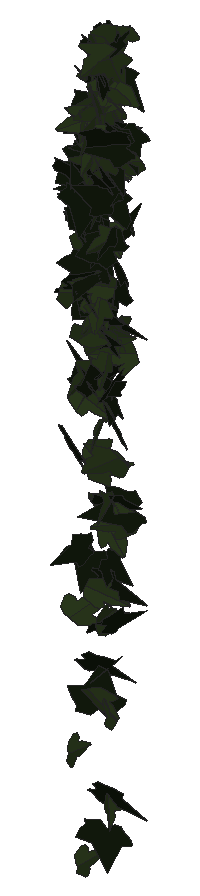
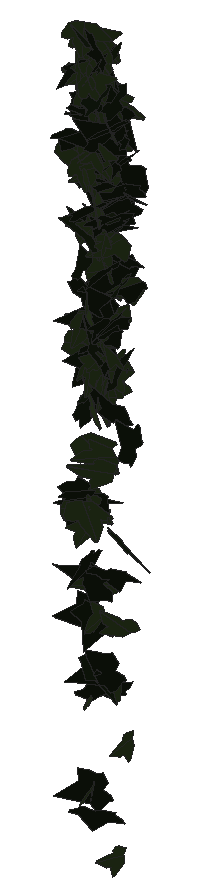
# SketchUp Ruby script. Lengths in inches.
U = 1.inch
M = Sketchup.active_model
def pt(a) = Geom::Point3d.new(a.map { |v| v * U })
def face(e, loops, mat)
  f = e.add_face(loops[0].map { |a| pt(a) })
  loops[1..].each { |l| e.add_face(l.map { |a| pt(a) }).erase! }
  f.material = f.back_material = mat if mat
  f
end
# faces: each face lists its corners as indices into pts; further lists are holes
def faces(e, pts, list, mat = nil) = list.each { |f| face(e, (f[0].is_a?(Array) ? f : [f]).map { |l| l.map { |i| pts[i] } }, mat) }
# xy, xz, yz: faces in a plane at the given z, y or x. An outline is a flat list of corners, or four numbers for a rectangle; further outlines are holes
def ring(l) = l.size == 4 ? [[l[0], l[1]], [l[2], l[1]], [l[2], l[3]], [l[0], l[3]]] : l.each_slice(2).to_a
def flat(e, list, mat, &to3) = list.each { |f| face(e, (f[0].is_a?(Array) ? f : [f]).map { |l| ring(l).map { |u, v| to3.(u, v) } }, mat) }
def xy(e, z, list, mat = nil) = flat(e, list, mat) { |x, y| [x, y, z] }
def xz(e, y, list, mat = nil) = flat(e, list, mat) { |x, z| [x, y, z] }
def yz(e, x, list, mat = nil) = flat(e, list, mat) { |y, z| [x, y, z] }
def lines(e, pts, list) = list.each { |a, b| e.add_line(pt(pts[a]), pt(pts[b])) }
# prism: a flat outline (further loops are holes) pulled along v
def prism(e, loops, v, mat = nil)
  f = face(e, loops, mat); d = Geom::Vector3d.new(v.map { |x| x * U })
  f.pushpull(f.normal.samedirection?(d) ? d.length : -d.length)
end
def box(e, o, s, mat = nil) = prism(e, [[o, [o[0] + s[0], o[1], o[2]], [o[0] + s[0], o[1] + s[1], o[2]], [o[0], o[1] + s[1], o[2]]]], [0, 0, s[2]], mat)
def at(x, y, z, deg = 0) = Geom::Transformation.translation(pt([x, y, z])) * Geom::Transformation.rotation(ORIGIN, Z_AXIS, deg.degrees)
def axes(o, x, y, z) = Geom::Transformation.new([*x, 0, *y, 0, *z, 0, *pt(o).to_a, 1])
def part(name) = M.definitions.add(name)
# library, detail: a bought-in or finely detailed component or shape, given as its bounding box
def library(name, o, s) = part(name).tap { |d| box(d.entities, o, s) }
def detail(e, o, s) = box(e.add_group.entities, o, s)
def put(e, d, t, mat = nil) = e.add_instance(d, t).tap { |i| i.material = mat if mat }
def group(e, t, mat = nil) = e.add_group.tap { |g| g.transformation = t; g.material = mat if mat }.entities
root = M.entities
M.materials.add("1026 AP 7946 SUNNY SIDE UP").color = [254, 231, 186]
M.materials.add("efeu1").color = [18, 25, 13]
M.materials.add("efeu2").color = [43, 57, 29]
c1 = part("ivyleaf_10")
p = [[0,0.5,-0.03],[-0.0625,2.02,-0.43],[-0.19,2.01,-0.46],[-0.54,1.05,-0.29],[-0.52,0.625,-0.18],[-0.83,0.76,-0.28],
  [-1.16,0.64,-0.33],[-1.15,0.33,-0.24],[-0.77,-0.39,0.02],[-0.3,-0.51,0.16],[0.04,-0.48,0.23],[-0.02,2.01,-0.4375],
  [-0.06,2.01,-0.43],[0.04,-0.49,0.23],[0.67,-0.49,0.14],[1.38,0.36,-0.2],[1.375,0.51,-0.24],[0.81,0.65,-0.19],
  [0.62,0.59,-0.15],[0.6,1.09,-0.28],[0.5,1.23,-0.31]]
faces(c1.entities,p,[[0,1,2,3,4,5,6,7,8,9,10],[11,12,0,13,14,15,16,17,18,19,20]],"efeu2")
c2 = part("ivyleaf_9")
p = [[1.54,2.16,1.25],[1.36,2.04,1.19],[-0.21,0.99,0.68],[-0.71,1.11,0.82],[-0.85,0.86,0.67],[-0.8,0.17,0.21],
  [-0.9,-0.01,0.1],[-0.67,-0.16,-0.02],[-0.08,-0.08,-0.05],[-0.03,-0.6,-0.4],[0.65,-0.88,-0.66],[0.83,-0.6,-0.49],
  [1.29,-0.42,-0.43],[1.8125,-0.07,-0.26],[1.21,0.44,0.15]]
faces(c2.entities,p,[[0,1,2,3,4,5,6,7,8,9,10,11,12,13,14]],"efeu1")
put(root,c1,axes([111.49,212.18,255.23],[0.26349,0.05357,-0.16919],[0.22588,0.08462,0.1796],[0.15168,-0.21907,0.02645]),"1026 AP 7946 SUNNY SIDE UP")
put(root,c2,axes([111.56,212.58,265.79],[-0.01777,-0.25367,-0.01098],[0.00914,0.00897,-0.26147],[0.39902,-0.0115,0.0055]),"1026 AP 7946 SUNNY SIDE UP")
put(root,c2,axes([111.58,212.3125,264.45],[-0.15826,-0.2049,-0.12442],[0.09307,0.10414,-0.23447],[0.36127,-0.11658,0.0059]),"1026 AP 7946 SUNNY SIDE UP")
put(root,c2,axes([111.5,212.4,265.18],[0.21603,-0.20442,-0.0599],[-0.03502,0.05362,-0.25316],[0.33184,0.13874,0.01228]),"1026 AP 7946 SUNNY SIDE UP")
put(root,c1,axes([111.69,212.07,264.54],[0.1941,-0.22333,0.03277],[0.00495,-0.03599,-0.26266],[0.35495,0.12263,-0.01426]),"1026 AP 7946 SUNNY SIDE UP")
put(root,c1,axes([111.73,212.0625,265.4],[-0.09146,0.18682,0.15912],[-0.11423,0.13697,-0.19943],[-0.36252,-0.09029,0.02269]),"1026 AP 7946 SUNNY SIDE UP")
put(root,c2,axes([111.5,212.48,259.78],[-0.1363,0.1013,0.21327],[0.24989,-0.13307,0.13523],[0.26134,0.18007,-0.01808]),"1026 AP 7946 SUNNY SIDE UP")
put(root,c2,axes([111.5625,212.44,261.74],[0.14333,-0.20924,-0.0936],[-0.06701,0.0792,-0.23455],[0.35162,0.10039,-0.00654]),"1026 AP 7946 SUNNY SIDE UP")
put(root,c2,axes([111.55,212.14,263.63],[0.15097,-0.22676,-0.03682],[-0.04058,0.02643,-0.25316],[0.35836,0.09852,-0.01316]),"1026 AP 7946 SUNNY SIDE UP")
put(root,c2,axes([111.43,211.99,258.95],[0.22206,-0.06541,-0.22293],[0.32923,-0.05721,0.15852],[-0.13255,-0.25167,0.02026]),"1026 AP 7946 SUNNY SIDE UP")
put(root,c2,axes([111.45,212.45,266.36],[0.29605,-0.16673,0.0648],[0.05532,-0.05632,-0.25873],[0.27523,0.19067,-0.0177]),"1026 AP 7946 SUNNY SIDE UP")
put(root,c2,axes([111.75,212.18,263.86],[0.31124,-0.00117,0.1752],[-0.26329,0.04437,0.20134],[-0.04685,-0.25717,0.03239]),"1026 AP 7946 SUNNY SIDE UP")
put(root,c2,axes([111.6,212.4375,261.6875],[0.00784,-0.19578,-0.15333],[-0.00771,0.14765,-0.20089],[0.38557,0.00693,-0.0009]),"1026 AP 7946 SUNNY SIDE UP")
put(root,c1,axes([111.9,212.58,265.2],[-0.34377,-0.00563,0.1266],[-0.18522,-0.0629,-0.21917],[0.05595,-0.2428,0.05232]),"1026 AP 7946 SUNNY SIDE UP")
put(root,c2,axes([111.625,211.9375,264.7],[0.44384,0.05371,-0.09486],[-0.13287,-0.04753,-0.29473],[-0.10285,0.29318,-0.02859]),"1026 AP 7946 SUNNY SIDE UP")
put(root,c1,axes([111.57,211.8,262.16],[-0.03675,-0.05095,-0.23565],[0.23229,0.17488,-0.05473],[0.28549,-0.14885,0.0142]),"1026 AP 7946 SUNNY SIDE UP")
put(root,c2,axes([111.72,212.41,256.45],[-0.29436,-0.1468,-0.06734],[0.09721,0.02546,-0.24427],[0.23266,-0.19637,0.01686]),"1026 AP 7946 SUNNY SIDE UP")
put(root,c2,axes([111.6875,212.21,264.8],[-0.09378,-0.20137,0.14095],[-0.05911,-0.13274,-0.21713],[0.37924,-0.07048,0.00101]),"1026 AP 7946 SUNNY SIDE UP")
put(root,c1,axes([111.72,212.38,265.78],[0.18876,-0.21054,0.07497],[0.04092,-0.07021,-0.2498],[0.3485,0.12228,-0.01127]),"1026 AP 7946 SUNNY SIDE UP")
put(root,c2,axes([111.95,211.9,256.875],[-0.31961,0.12959,-0.02596],[0.01723,-0.0309,-0.24765],[-0.20709,-0.20257,0.01947]),"1026 AP 7946 SUNNY SIDE UP")
put(root,c2,axes([111.64,212.58,262.82],[0.07735,-0.23071,-0.0778],[-0.02575,0.07239,-0.24259],[0.38021,0.05184,-0.0006]),"1026 AP 7946 SUNNY SIDE UP")
put(root,c1,axes([111.83,212.25,266.01],[-0.07473,-0.23429,0.07325],[-0.00508,-0.07317,-0.24645],[0.38557,-0.04637,0.01095]),"1026 AP 7946 SUNNY SIDE UP")
put(root,c1,axes([111.74,211.75,252.61],[-0.00129,-0.04435,-0.2514],[0.09781,0.23594,-0.04306],[0.37714,-0.06134,0.01031]),"1026 AP 7946 SUNNY SIDE UP")
put(root,c1,axes([111.6875,212.46,261.11],[0.34374,-0.11681,0.10042],[0.11864,-0.06627,-0.25478],[0.2085,0.23028,-0.02058]),"1026 AP 7946 SUNNY SIDE UP")
put(root,c2,axes([111.67,212.35,263.78],[-0.05512,-0.23077,-0.12773],[0.04427,0.11972,-0.2396],[0.40855,-0.04411,0.00873]),"1026 AP 7946 SUNNY SIDE UP")
put(root,c2,axes([112,212.04,265.81],[0.11588,0.09421,-0.22902],[-0.28417,-0.13344,-0.12047],[-0.25292,0.19309,0.03042]),"1026 AP 7946 SUNNY SIDE UP")
put(root,c2,axes([111.93,212.14,260.21],[0.07343,-0.2493,0.13933],[-0.02013,0.13651,0.26185],[-0.44659,-0.04714,0.0111]),"1026 AP 7946 SUNNY SIDE UP")
put(root,c2,axes([111.5625,212.35,265.27],[0.14322,-0.14456,0.18881],[0.15484,-0.15555,-0.17693],[0.3339,0.13414,0.00106]),"1026 AP 7946 SUNNY SIDE UP")
put(root,c2,axes([111.7,212.4,265.43],[-0.07135,-0.02984,0.28062],[0.36249,0.14542,0.05679],[-0.23342,0.23495,0.00241]),"1026 AP 7946 SUNNY SIDE UP")
put(root,c1,axes([111.68,212.19,263.22],[-0.17067,-0.10762,-0.20235],[0.2606,0.10722,-0.15473],[0.23563,-0.19654,0.02456]),"1026 AP 7946 SUNNY SIDE UP")
put(root,c1,axes([111.8,212.07,260.42],[0.04402,-0.09335,0.29078],[0.12483,-0.27141,-0.10199],[0.4513,0.08418,-0.00015]),"1026 AP 7946 SUNNY SIDE UP")
put(root,c1,axes([112.03,211.96,265.89],[0.22377,0.05359,-0.2239],[-0.29814,-0.10871,-0.15593],[-0.18797,0.23623,-0.01922]),"1026 AP 7946 SUNNY SIDE UP")
put(root,c2,axes([111.76,212.02,264.05],[-0.06303,-0.24689,0.08918],[0.00151,-0.08913,-0.25777],[0.41212,-0.03743,0.01459]),"1026 AP 7946 SUNNY SIDE UP")
put(root,c2,axes([111.58,212.35,265.42],[0.21953,0.059,0.22804],[0.3316,0.06714,-0.15531],[-0.13939,0.25266,-0.01032]),"1026 AP 7946 SUNNY SIDE UP")
put(root,c1,axes([111.92,212.62,266.66],[-0.17471,-0.20305,0.11598],[-0.00404,-0.12495,-0.23313],[0.36593,-0.09832,0.0528]),"1026 AP 7946 SUNNY SIDE UP")
put(root,c2,axes([111.66,211.79,262.33],[0.26184,0.14155,0.21204],[0.26564,0.1171,-0.22396],[-0.28793,0.23675,-0.01379]),"1026 AP 7946 SUNNY SIDE UP")
put(root,c2,axes([111.79,212.38,267.13],[0.18853,-0.18165,-0.17069],[-0.14945,0.13452,-0.22339],[0.35536,0.15294,-0.00339]),"1026 AP 7946 SUNNY SIDE UP")
put(root,c2,axes([111.7,212.12,262.22],[0.17634,-0.23271,0.03459],[0.0087,-0.03604,-0.26611],[0.36991,0.11178,-0.01023]),"1026 AP 7946 SUNNY SIDE UP")
put(root,c1,axes([111.91,212.05,260.04],[0.00158,-0.22037,-0.1156],[0.03959,0.11047,-0.22515],[0.38594,-0.01043,0.02357]),"1026 AP 7946 SUNNY SIDE UP")
put(root,c2,axes([112.21,212.3,264.34],[-0.35931,0.03377,0.14084],[-0.21935,-0.02139,-0.23522],[-0.02805,-0.26533,0.0353]),"1026 AP 7946 SUNNY SIDE UP")
put(root,c2,axes([111.83,212.34,263.65],[-0.14994,-0.16841,0.16867],[0.04664,-0.18483,-0.17812],[0.36743,-0.04526,0.09144]),"1026 AP 7946 SUNNY SIDE UP")
put(root,c1,axes([111.9375,212.23,260.2],[-0.03129,-0.18796,-0.16403],[0.02492,0.15736,-0.1938],[0.38545,-0.02544,-0.00079]),"1026 AP 7946 SUNNY SIDE UP")
put(root,c1,axes([111.98,212.4375,264.14],[0.07847,-0.22179,-0.1088],[-0.03734,0.10162,-0.2336],[0.3836,0.05526,-0.00048]),"1026 AP 7946 SUNNY SIDE UP")
put(root,c2,axes([111.66,212.375,265.01],[0.35645,-0.09086,0.05928],[0.06862,-0.04627,-0.25044],[0.15504,0.22939,-0.02543]),"1026 AP 7946 SUNNY SIDE UP")
put(root,c1,axes([111.85,211.9,250.24],[0.01853,0.01717,-0.24859],[0.14718,0.22256,0.02232],[0.35093,-0.09425,0.00377]),"1026 AP 7946 SUNNY SIDE UP")
put(root,c1,axes([112,212.29,263.32],[-0.3098,0.11761,0.04413],[-0.08052,-0.0042,-0.23446],[-0.17919,-0.20144,0.02907]),"1026 AP 7946 SUNNY SIDE UP")
put(root,c1,axes([111.95,212.5,266.86],[-0.00906,-0.2231,0.14393],[0.03576,-0.14091,-0.22958],[0.41343,0.0073,0.02301]),"1026 AP 7946 SUNNY SIDE UP")
put(root,c1,axes([111.85,212.1,265.83],[0.03925,-0.1576,0.20933],[0.14963,-0.18494,-0.1602],[0.37684,0.08985,0.04181]),"1026 AP 7946 SUNNY SIDE UP")
put(root,c1,axes([111.98,212.26,266.07],[0.01259,-0.24051,0.0723],[-0.00702,-0.07171,-0.24824],[0.3945,0.0064,-0.00673]),"1026 AP 7946 SUNNY SIDE UP")
put(root,c1,axes([112.07,212.32,266.5],[-0.36898,-0.08384,0.08035],[-0.0935,-0.06401,-0.25401],[0.15447,-0.23901,0.03818]),"1026 AP 7946 SUNNY SIDE UP")
put(root,c2,axes([111.97,212,262.78],[-0.3273,-0.12048,-0.06705],[0.10244,0.01562,-0.24695],[0.18881,-0.21733,0.01776]),"1026 AP 7946 SUNNY SIDE UP")
put(root,c1,axes([111.86,212.37,267.23],[-0.29736,0.11937,-0.136],[0.13304,-0.11026,-0.22706],[-0.24711,-0.20301,0.04141]),"1026 AP 7946 SUNNY SIDE UP")
put(root,c2,axes([111.79,212.41,266.99],[0.0234,-0.21581,0.15369],[0.05971,-0.14731,-0.22248],[0.4093,0.03383,0.02367]),"1026 AP 7946 SUNNY SIDE UP")
put(root,c1,axes([111.75,212.29,262.65],[0.02285,-0.03083,0.26184],[0.32226,-0.15148,-0.03187],[0.24176,0.20483,0.01773]),"1026 AP 7946 SUNNY SIDE UP")
put(root,c1,axes([111.97,212.1,266.09],[-0.01819,-0.18153,-0.17931],[0.07071,0.16889,-0.18466],[0.38793,-0.0393,0.02525]),"1026 AP 7946 SUNNY SIDE UP")
put(root,c2,axes([112.2,212.01,266.86],[0.06598,-0.01153,-0.26858],[-0.40906,0.01821,-0.04387],[0.03118,0.26337,-0.00718]),"1026 AP 7946 SUNNY SIDE UP")
put(root,c2,axes([111.78,212.5625,266.33],[0.18005,-0.21772,0.07218],[0.02467,-0.07207,-0.2531],[0.35939,0.11402,-0.01879]),"1026 AP 7946 SUNNY SIDE UP")
put(root,c2,axes([111.75,212.23,254.3],[0.34168,0.03996,0.10675],[0.16355,0.00516,-0.22722],[-0.06026,0.24059,-0.01142]),"1026 AP 7946 SUNNY SIDE UP")
put(root,c1,axes([112.25,212.28,257.6],[0.04509,-0.03082,-0.25089],[-0.29906,0.15196,-0.04203],[0.24362,0.19225,-0.00515]),"1026 AP 7946 SUNNY SIDE UP")
put(root,c1,axes([111.87,212.53,259.59],[0.10718,-0.16184,-0.17592],[0.11955,-0.15208,0.17984],[-0.34899,-0.10181,0.00758]),"1026 AP 7946 SUNNY SIDE UP")
put(root,c1,axes([112.1,212.28,261.37],[-0.25316,-0.16535,-0.10622],[-0.11783,-0.06961,0.23729],[-0.282,0.17752,-0.00379]),"1026 AP 7946 SUNNY SIDE UP")
put(root,c1,axes([111.93,212.43,260.8],[0.04215,0.19016,0.15565],[0.05133,0.14671,-0.19674],[-0.37736,0.0412,-0.00938]),"1026 AP 7946 SUNNY SIDE UP")
put(root,c2,axes([112.26,212.43,261.97],[0.01527,-0.00009,0.25561],[-0.23078,0.20021,0.00716],[-0.31457,-0.14688,0.00715]),"1026 AP 7946 SUNNY SIDE UP")
put(root,c1,axes([112.09,212.1875,255.24],[0.0297,-0.00295,0.27529],[-0.14059,0.2524,0.01086],[-0.39602,-0.08983,0.01679]),"1026 AP 7946 SUNNY SIDE UP")
put(root,c2,axes([111.93,212.35,260.9],[0.03684,0.20856,0.1334],[-0.04978,-0.12523,0.21493],[0.3818,-0.03645,0.01515]),"1026 AP 7946 SUNNY SIDE UP")
put(root,c1,axes([112.27,212.08,262.38],[-0.03316,-0.04049,-0.27367],[-0.34489,-0.15094,0.04079],[-0.24347,0.21933,-0.02051]),"1026 AP 7946 SUNNY SIDE UP")
put(root,c1,axes([112.07,212.43,260.55],[-0.03924,-0.20265,-0.1391],[0.02828,0.13267,-0.20956],[0.38085,-0.03073,0.00123]),"1026 AP 7946 SUNNY SIDE UP")
put(root,c1,axes([112.21,212.48,257.61],[-0.39451,-0.04793,0.10706],[-0.15128,-0.04845,-0.26192],[0.09816,-0.26732,0.02661]),"1026 AP 7946 SUNNY SIDE UP")
put(root,c1,axes([112.09,212.48,264.68],[0.01884,-0.2399,-0.02471],[-0.0018,0.02259,-0.24731],[0.37888,0.01203,0.00005]),"1026 AP 7946 SUNNY SIDE UP")
put(root,c2,axes([112.21,212.22,254.3],[-0.14652,0.21919,-0.06287],[0.02194,-0.06166,-0.24547],[-0.35763,-0.09358,0.0107]),"1026 AP 7946 SUNNY SIDE UP")
put(root,c1,axes([111.99,212.34,264.42],[-0.39469,0.00831,0.09381],[0.14371,0.02071,0.25783],[0.00115,0.2662,-0.02142]),"1026 AP 7946 SUNNY SIDE UP")
put(root,c1,axes([112.04,212.03,265.73],[0.11508,-0.22307,0.1667],[0.07723,-0.15551,-0.24276],[0.42757,0.08813,-0.00102]),"1026 AP 7946 SUNNY SIDE UP")
put(root,c1,axes([112.1875,211.98,265],[-0.32008,-0.15967,0.07406],[-0.06661,-0.06347,-0.26585],[0.26776,-0.20665,0.02239]),"1026 AP 7946 SUNNY SIDE UP")
put(root,c1,axes([111.97,211.84,261.31],[-0.17736,-0.15113,0.16379],[0.11863,0.14217,0.19415],[-0.32492,0.1344,-0.01852]),"1026 AP 7946 SUNNY SIDE UP")
put(root,c1,axes([112.06,212.04,265.21],[-0.05317,-0.15176,0.21399],[0.09238,-0.20937,-0.14834],[0.39494,0.02854,0.06351]),"1026 AP 7946 SUNNY SIDE UP")
put(root,c2,axes([111.87,212.58,267.4],[-0.09084,-0.02861,-0.26183],[0.40162,-0.01635,-0.05804],[-0.01526,-0.25997,0.03092]),"1026 AP 7946 SUNNY SIDE UP")
put(root,c1,axes([112.22,212.02,261.41],[-0.27817,-0.14677,0.10103],[-0.09895,-0.07854,-0.23648],[0.2601,-0.18684,0.01808]),"1026 AP 7946 SUNNY SIDE UP")
put(root,c1,axes([112.14,212.57,264.87],[-0.19531,-0.21729,-0.00115],[0.0135,-0.00504,-0.25767],[0.34139,-0.12411,0.00953]),"1026 AP 7946 SUNNY SIDE UP")
put(root,c1,axes([112.05,212.23,263.98],[0.11376,-0.15594,0.16815],[0.09081,-0.15387,-0.17776],[0.34419,0.09214,-0.00868]),"1026 AP 7946 SUNNY SIDE UP")
put(root,c1,axes([111.86,212.25,258.73],[0.09051,0.06408,0.23441],[0.25887,0.15666,-0.08758],[-0.26596,0.17429,-0.00547]),"1026 AP 7946 SUNNY SIDE UP")
put(root,c2,axes([111.85,212.4,266.21],[0.07976,-0.13098,0.21705],[0.17116,-0.18233,-0.14433],[0.35163,0.11846,0.02102]),"1026 AP 7946 SUNNY SIDE UP")
put(root,c2,axes([111.97,212.08,261.3125],[0.37732,0.02796,-0.02469],[-0.03382,-0.02313,-0.24813],[-0.04721,0.24006,-0.0196]),"1026 AP 7946 SUNNY SIDE UP")
put(root,c1,axes([112.37,212.14,258.75],[-0.29058,-0.06675,0.2051],[-0.27424,-0.09979,-0.20145],[0.18488,-0.25294,0.02354]),"1026 AP 7946 SUNNY SIDE UP")
put(root,c2,axes([112.15,212.27,265.32],[-0.33998,0.00625,-0.13645],[0.2046,-0.03915,-0.22089],[-0.04045,-0.25054,0.02962]),"1026 AP 7946 SUNNY SIDE UP")
put(root,c1,axes([111.93,212.38,264.74],[-0.0933,-0.15326,-0.19128],[0.28614,0.09546,-0.14119],[0.24624,-0.16899,0.09159]),"1026 AP 7946 SUNNY SIDE UP")
put(root,c1,axes([112.27,212.16,267.23],[-0.21641,-0.17201,0.19573],[-0.11561,-0.18123,-0.22381],[0.38725,-0.15023,0.04257]),"1026 AP 7946 SUNNY SIDE UP")
put(root,c2,axes([111.95,212.55,264.01],[0.06847,-0.22172,-0.11837],[0.02687,0.11775,-0.22924],[0.39084,0.03075,0.0365]),"1026 AP 7946 SUNNY SIDE UP")
put(root,c1,axes([112.125,211.93,266.39],[-0.23878,0.20286,0.00951],[-0.02943,-0.00394,-0.26047],[-0.31787,-0.15202,0.01697]),"1026 AP 7946 SUNNY SIDE UP")
put(root,c2,axes([112.16,212.01,253.58],[-0.31542,-0.08672,0.19401],[0.25026,0.10458,0.22429],[-0.21001,0.25486,-0.02411]),"1026 AP 7946 SUNNY SIDE UP")
put(root,c2,axes([112.13,212.16,255.27],[0.13304,0.22066,0.06879],[0.05305,0.05717,-0.24288],[-0.35803,0.09047,-0.01042]),"1026 AP 7946 SUNNY SIDE UP")
put(root,c2,axes([112.45,212.01,263.26],[-0.35762,-0.12018,-0.11605],[-0.17552,-0.02721,0.26351],[-0.18947,0.25204,-0.02506]),"1026 AP 7946 SUNNY SIDE UP")
put(root,c2,axes([111.82,212.3,261.64],[0.36177,-0.03212,0.13157],[0.19483,-0.03537,-0.23898],[0.07096,0.26085,-0.01463]),"1026 AP 7946 SUNNY SIDE UP")
put(root,c2,axes([111.99,212.35,265.12],[0.10688,-0.23908,-0.07997],[-0.02401,0.07493,-0.25556],[0.39386,0.06944,0.00612]),"1026 AP 7946 SUNNY SIDE UP")
put(root,c1,axes([111.91,212.24,258.37],[0.07759,0.01388,-0.26692],[0.33103,0.15215,0.05058],[0.23869,-0.21553,0.01662]),"1026 AP 7946 SUNNY SIDE UP")
put(root,c1,axes([112.23,212.125,261.86],[-0.07385,-0.20198,0.18652],[-0.0452,-0.18017,-0.21446],[0.42532,-0.05422,0.0096]),"1026 AP 7946 SUNNY SIDE UP")
put(root,c1,axes([112,212.61,261.79],[0.09887,-0.03927,0.24002],[0.22759,-0.18444,-0.07328],[0.29408,0.15594,-0.02398]),"1026 AP 7946 SUNNY SIDE UP")
put(root,c2,axes([112.33,212.13,264.16],[-0.01628,0.01664,0.27149],[-0.34139,-0.15048,0.00013],[0.23605,-0.21648,0.0189]),"1026 AP 7946 SUNNY SIDE UP")
put(root,c2,axes([111.92,212.18,261.72],[0.08689,-0.04807,0.24498],[0.20126,-0.20174,-0.07375],[0.32457,0.13797,-0.01985]),"1026 AP 7946 SUNNY SIDE UP")
put(root,c1,axes([111.92,211.86,260.06],[0.17084,0.07687,0.21732],[0.31015,0.07826,-0.13386],[-0.16728,0.2236,-0.02624]),"1026 AP 7946 SUNNY SIDE UP")
put(root,c2,axes([112.2,211.97,260.21],[0.27436,0.07539,0.17121],[-0.25506,-0.03999,0.19441],[0.13013,-0.23733,0.02006]),"1026 AP 7946 SUNNY SIDE UP")
put(root,c1,axes([112.24,212.45,267.57],[-0.3289,-0.146,-0.00522],[0.02961,-0.01962,-0.26144],[0.22776,-0.20829,0.02646]),"1026 AP 7946 SUNNY SIDE UP")
put(root,c2,axes([112.41,212.36,267.47],[-0.28647,0.17662,-0.02994],[0.01399,-0.03391,-0.26095],[-0.28137,-0.18151,0.01751]),"1026 AP 7946 SUNNY SIDE UP")
put(root,c1,axes([112.26,212.04,266.05],[-0.30034,-0.23882,-0.01946],[0.04106,0.00152,-0.3144],[0.37429,-0.1918,0.01888]),"1026 AP 7946 SUNNY SIDE UP")
put(root,c1,axes([112.1,211.96,253.83],[-0.29101,-0.01477,-0.14565],[0.2233,-0.01293,-0.19031],[0.00606,-0.23249,0.01847]),"1026 AP 7946 SUNNY SIDE UP")
put(root,c2,axes([112.11,212.35,265.08],[0.04439,-0.25416,-0.05049],[0.00088,0.04791,-0.2631],[0.40658,0.02765,0.00608]),"1026 AP 7946 SUNNY SIDE UP")
put(root,c1,axes([112.19,212.28,257.76],[0.05761,-0.08989,0.22912],[0.13122,-0.20671,-0.10121],[0.35443,0.09114,0.00023]),"1026 AP 7946 SUNNY SIDE UP")
put(root,c2,axes([112.27,212.15,263.54],[-0.29978,0.02955,-0.16515],[0.23577,-0.06564,-0.19634],[-0.10122,-0.2404,0.03178]),"1026 AP 7946 SUNNY SIDE UP")
put(root,c2,axes([112.2,212.25,256.53],[0.12854,-0.10366,-0.20948],[-0.1577,0.17702,-0.13386],[0.32147,0.12829,0.01809]),"1026 AP 7946 SUNNY SIDE UP")
put(root,c1,axes([112.23,211.95,259.51],[0.15653,-0.19989,0.11283],[0.07577,-0.09962,-0.23063],[0.35117,0.11059,-0.00053]),"1026 AP 7946 SUNNY SIDE UP")
put(root,c1,axes([112.01,212.08,255.93],[0.07853,0.06296,0.23563],[0.28628,0.13911,-0.07971],[-0.23829,0.18787,-0.01812]),"1026 AP 7946 SUNNY SIDE UP")
put(root,c2,axes([112.22,211.96,260.49],[-0.04821,0.20251,-0.17994],[-0.06468,0.17131,0.21167],[0.41669,0.05002,0.01204]),"1026 AP 7946 SUNNY SIDE UP")
put(root,c1,axes([112.52,212.375,260.9375],[0.08292,0.00101,-0.27126],[-0.35351,-0.13963,-0.04775],[-0.21555,0.22939,-0.02603]),"1026 AP 7946 SUNNY SIDE UP")
put(root,c1,axes([112.17,212.29,263.43],[0.20166,0.18652,0.06269],[0.07945,0.03755,-0.23209],[-0.29757,0.13643,-0.01948]),"1026 AP 7946 SUNNY SIDE UP")
put(root,c1,axes([112.13,212.29,266.71],[-0.18187,-0.1564,-0.16661],[0.26763,0.05672,-0.18258],[0.22982,-0.18982,0.08077]),"1026 AP 7946 SUNNY SIDE UP")
put(root,c1,axes([112.3,212.1,263.38],[0.00609,-0.02855,0.2571],[0.04809,-0.24784,-0.03113],[0.39229,0.03083,-0.00018]),"1026 AP 7946 SUNNY SIDE UP")
put(root,c2,axes([112.21,212.25,257.83],[0.34294,0.10515,-0.02508],[-0.0232,-0.02668,-0.24894],[-0.16834,0.2179,-0.01679]),"1026 AP 7946 SUNNY SIDE UP")
put(root,c2,axes([112.17,212.3,259.98],[0.00659,-0.19516,0.18616],[0.01966,-0.18149,-0.20206],[0.41894,0.01159,0.00655]),"1026 AP 7946 SUNNY SIDE UP")
put(root,c1,axes([112.22,211.9,262.07],[0.35625,-0.08504,0.06961],[0.08877,-0.04263,-0.24876],[0.14646,0.23269,-0.01855]),"1026 AP 7946 SUNNY SIDE UP")
put(root,c1,axes([112.29,212.37,261.4375],[-0.11364,-0.19325,-0.14285],[0.09334,0.1245,-0.21158],[0.36113,-0.09299,0.00973]),"1026 AP 7946 SUNNY SIDE UP")
put(root,c1,axes([112.22,212.27,257.19],[0.1334,0.23441,0.08072],[0.04982,0.07042,-0.25634],[-0.38476,0.09039,-0.00521]),"1026 AP 7946 SUNNY SIDE UP")
put(root,c1,axes([112.09,212.32,261.15],[-0.19917,-0.02997,0.20787],[0.30988,0.04411,0.13434],[-0.08383,0.23427,0.00274]),"1026 AP 7946 SUNNY SIDE UP")
put(root,c1,axes([112.27,212.11,266.44],[-0.37802,0.01035,-0.0781],[0.11452,-0.04628,-0.24452],[-0.03717,-0.24781,0.04091]),"1026 AP 7946 SUNNY SIDE UP")
put(root,c2,axes([112.32,212.28,263.28],[-0.2125,0.24011,-0.05443],[-0.02625,0.05275,0.28393],[0.38616,0.13572,-0.01065]),"1026 AP 7946 SUNNY SIDE UP")
put(root,c1,axes([112.35,212.31,266.75],[-0.03462,-0.20921,-0.14626],[0.03289,0.13932,-0.21584],[0.39515,-0.02993,0.00515]),"1026 AP 7946 SUNNY SIDE UP")
put(root,c2,axes([112.19,212.53,262.64],[0.01684,-0.13978,0.21086],[0.02779,-0.20471,-0.14562],[0.38977,0.02064,0.00127]),"1026 AP 7946 SUNNY SIDE UP")
put(root,c2,axes([111.99,212.25,256.05],[0.1823,-0.03133,-0.23766],[0.33636,0.11558,0.09533],[0.14376,-0.23069,0.07832]),"1026 AP 7946 SUNNY SIDE UP")
put(root,c2,axes([112.0625,212.18,251.6875],[0.3489,-0.01749,0.10491],[0.15487,-0.03788,-0.22779],[0.04963,0.24123,-0.02671]),"1026 AP 7946 SUNNY SIDE UP")
put(root,c2,axes([112.12,212.05,264.8],[0.0429,-0.09422,0.26556],[0.12027,-0.24674,-0.10248],[0.41528,0.08119,0.00224]),"1026 AP 7946 SUNNY SIDE UP")
put(root,c2,axes([112.49,211.83,265.78],[0.10041,0.18244,-0.1682],[-0.1175,-0.14727,-0.19925],[-0.36774,0.09687,0.01774]),"1026 AP 7946 SUNNY SIDE UP")
put(root,c1,axes([112.61,212.43,264.98],[-0.14866,-0.05881,0.23396],[-0.27984,-0.1421,-0.1149],[0.24111,-0.20119,0.0109]),"1026 AP 7946 SUNNY SIDE UP")
put(root,c2,axes([112.45,211.98,260.37],[-0.10761,0.10434,-0.24779],[-0.21984,0.19649,0.12962],[0.34975,0.15561,0.00524]),"1026 AP 7946 SUNNY SIDE UP")
put(root,c1,axes([112.32,212.13,251.59],[-0.02314,0.21585,-0.10847],[0.00851,-0.10639,-0.2235],[-0.37838,-0.01559,0.00161]),"1026 AP 7946 SUNNY SIDE UP")
put(root,c2,axes([112.61,212.4375,257.66],[-0.29885,-0.0718,0.19513],[-0.24823,-0.11112,-0.20679],[0.20054,-0.24455,0.03482]),"1026 AP 7946 SUNNY SIDE UP")
put(root,c1,axes([112.4,212.18,266.56],[0.40958,0.06232,-0.07723],[-0.10562,-0.04165,-0.27505],[-0.11168,0.26793,-0.0231]),"1026 AP 7946 SUNNY SIDE UP")
put(root,c1,axes([112.39,212.125,253.375],[-0.14264,0.20862,0.09575],[0.0615,-0.08304,0.23386],[0.35304,0.09876,-0.00206]),"1026 AP 7946 SUNNY SIDE UP")
put(root,c1,axes([112.32,211.98,260.91],[0.29336,-0.14732,0.1034],[0.10724,-0.07655,-0.24476],[0.25978,0.19796,-0.01572]),"1026 AP 7946 SUNNY SIDE UP")
put(root,c2,axes([112.48,212.22,259.32],[0.11143,-0.21266,0.10299],[-0.01691,0.10263,0.23058],[-0.36992,-0.06875,0.02049]),"1026 AP 7946 SUNNY SIDE UP")
put(root,c1,axes([112.58,212.36,257.42],[-0.04192,-0.00052,0.2849],[-0.16129,-0.258,-0.01219],[0.40383,-0.10309,0.0247]),"1026 AP 7946 SUNNY SIDE UP")
put(root,c2,axes([112.35,212,251.05],[-0.22701,-0.16877,-0.11023],[0.13182,0.06738,-0.22766],[0.28435,-0.16598,0.01754]),"1026 AP 7946 SUNNY SIDE UP")
put(root,c2,axes([112.3,212.55,265.45],[-0.08296,-0.21249,-0.13109],[0.05193,0.12166,-0.22483],[0.38499,-0.0622,0.00208]),"1026 AP 7946 SUNNY SIDE UP")
put(root,c2,axes([112.28,212.16,255.26],[0.11659,0.07362,0.22991],[0.24337,0.16021,-0.10668],[-0.27723,0.17161,0.00303]),"1026 AP 7946 SUNNY SIDE UP")
put(root,c2,axes([112.71,212.05,265.48],[-0.33715,0.0153,0.14367],[-0.22044,-0.01931,-0.22012],[-0.00353,-0.255,0.02379]),"1026 AP 7946 SUNNY SIDE UP")
put(root,c2,axes([112.27,212.31,266.75],[0.02876,-0.17057,-0.19242],[0.0286,0.18671,-0.17363],[0.39557,-0.0011,0.02655]),"1026 AP 7946 SUNNY SIDE UP")
put(root,c1,axes([112.42,212.08,267.14],[-0.2059,-0.2192,-0.10431],[0.1025,0.07735,-0.26212],[0.36472,-0.14548,0.01478]),"1026 AP 7946 SUNNY SIDE UP")
